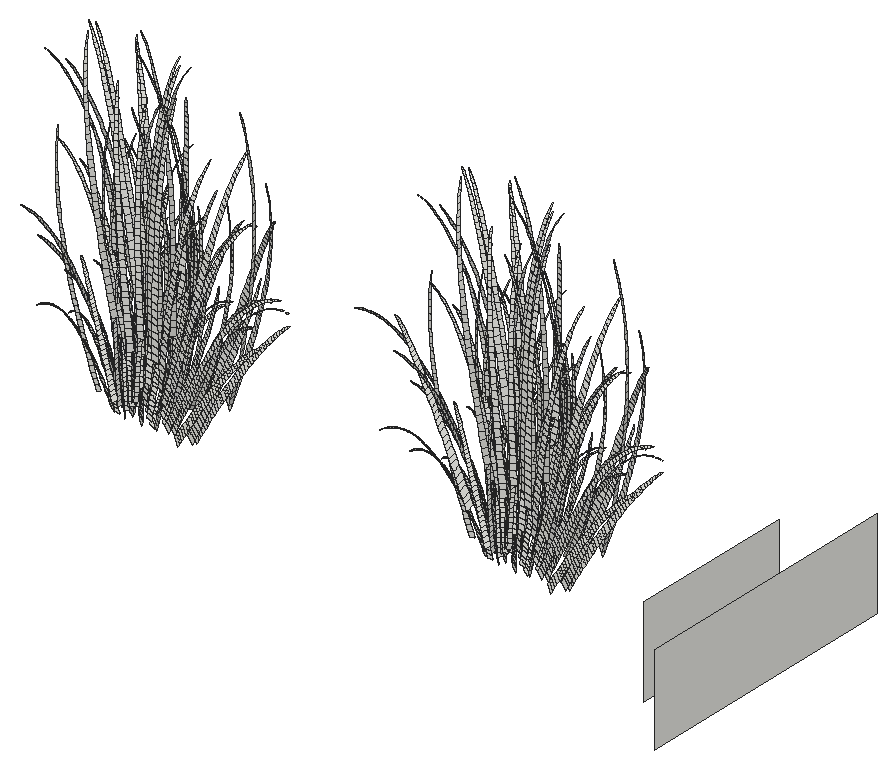
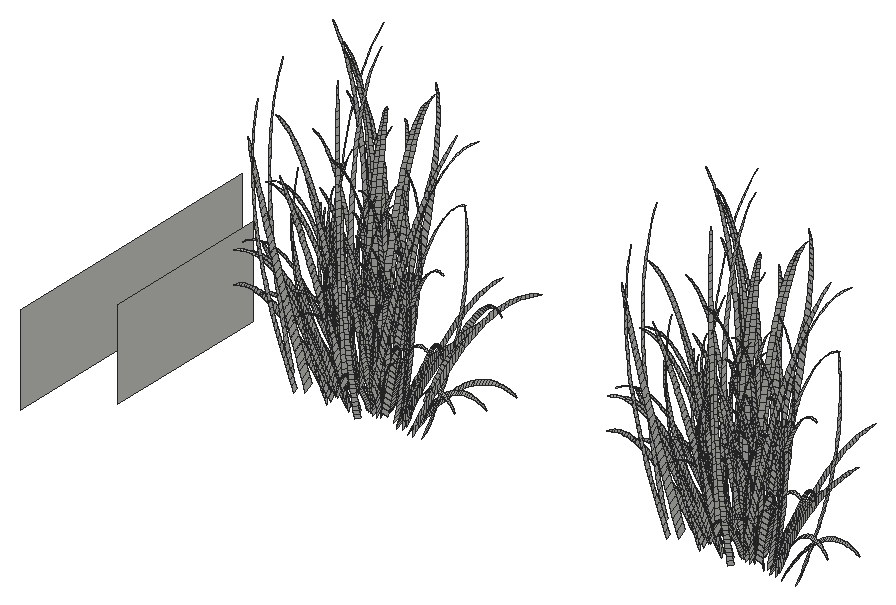
# SketchUp Ruby script. Lengths in inches.
U = 1.inch
M = Sketchup.active_model
def pt(a) = Geom::Point3d.new(a.map { |v| v * U })
def face(e, loops, mat)
  f = e.add_face(loops[0].map { |a| pt(a) })
  loops[1..].each { |l| e.add_face(l.map { |a| pt(a) }).erase! }
  f.material = f.back_material = mat if mat
  f
end
# faces: each face lists its corners as indices into pts; further lists are holes
def faces(e, pts, list, mat = nil) = list.each { |f| face(e, (f[0].is_a?(Array) ? f : [f]).map { |l| l.map { |i| pts[i] } }, mat) }
# xy, xz, yz: faces in a plane at the given z, y or x. An outline is a flat list of corners, or four numbers for a rectangle; further outlines are holes
def ring(l) = l.size == 4 ? [[l[0], l[1]], [l[2], l[1]], [l[2], l[3]], [l[0], l[3]]] : l.each_slice(2).to_a
def flat(e, list, mat, &to3) = list.each { |f| face(e, (f[0].is_a?(Array) ? f : [f]).map { |l| ring(l).map { |u, v| to3.(u, v) } }, mat) }
def xy(e, z, list, mat = nil) = flat(e, list, mat) { |x, y| [x, y, z] }
def xz(e, y, list, mat = nil) = flat(e, list, mat) { |x, z| [x, y, z] }
def yz(e, x, list, mat = nil) = flat(e, list, mat) { |y, z| [x, y, z] }
def lines(e, pts, list) = list.each { |a, b| e.add_line(pt(pts[a]), pt(pts[b])) }
# prism: a flat outline (further loops are holes) pulled along v
def prism(e, loops, v, mat = nil)
  f = face(e, loops, mat); d = Geom::Vector3d.new(v.map { |x| x * U })
  f.pushpull(f.normal.samedirection?(d) ? d.length : -d.length)
end
def box(e, o, s, mat = nil) = prism(e, [[o, [o[0] + s[0], o[1], o[2]], [o[0] + s[0], o[1] + s[1], o[2]], [o[0], o[1] + s[1], o[2]]]], [0, 0, s[2]], mat)
def at(x, y, z, deg = 0) = Geom::Transformation.translation(pt([x, y, z])) * Geom::Transformation.rotation(ORIGIN, Z_AXIS, deg.degrees)
def axes(o, x, y, z) = Geom::Transformation.new([*x, 0, *y, 0, *z, 0, *pt(o).to_a, 1])
def part(name) = M.definitions.add(name)
# library, detail: a bought-in or finely detailed component or shape, given as its bounding box
def library(name, o, s) = part(name).tap { |d| box(d.entities, o, s) }
def detail(e, o, s) = box(e.add_group.entities, o, s)
def put(e, d, t, mat = nil) = e.add_instance(d, t).tap { |i| i.material = mat if mat }
def group(e, t, mat = nil) = e.add_group.tap { |g| g.transformation = t; g.material = mat if mat }.entities
root = M.entities
c1 = part("fur_instance\#8")
p = [[-0.25,1.49,0.03],[0.25,-1.49,-0.03],[0.44,-1.47,1.51],[-0.05,1.47,1.57],[0.65,-1.44,3.05],[0.16,1.45,3.11],
  [0.86,-1.42,4.59],[0.38,1.44,4.65],[1.1,-1.39,6.13],[0.62,1.43,6.18],[1.34,-1.35,7.66],[0.875,1.42,7.72],
  [1.6,-1.32,9.19],[1.14,1.41,9.25],[1.88,-1.28,10.72],[1.43,1.41,10.78],[2.18,-1.24,12.25],[1.73,1.41,12.3],
  [2.49,-1.19,13.77],[2.05,1.41,13.82],[2.83,-1.15,15.29],[2.4,1.41,15.34],[3.18,-1.09,16.8],[2.76,1.42,16.85],
  [3.56,-1.03,18.31],[3.14,1.43,18.35],[3.96,-0.97,19.81],[3.55,1.44,19.85],[4.38,-0.91,21.3],[3.99,1.46,21.35],
  [4.84,-0.83,22.78],[4.45,1.48,22.83],[5.32,-0.76,24.26],[4.93,1.51,24.31],[5.82,-0.67,25.73],[5.45,1.54,25.77],
  [6.36,-0.59,27.18],[6,1.57,27.23],[6.93,-0.49,28.625],[6.58,1.61,28.67],[7.54,-0.39,30.05],[7.19,1.66,30.1],
  [8.18,-0.28,31.47],[7.84,1.71,31.51],[8.85,-0.16,32.86],[8.53,1.77,32.9],[9.57,-0.04,34.24],[9.25,1.83,34.27],
  [10.32,0.09,35.59],[10.02,1.9,35.625],[11.12,0.23,36.92],[10.82,1.97,36.95],[11.95,0.38,38.22],[11.67,2.06,38.25],
  [12.84,0.54,39.49],[12.57,2.14,39.52],[13.76,0.71,40.73],[13.51,2.24,40.76],[14.73,0.89,41.93],[14.49,2.34,41.95],
  [15.75,1.08,43.09],[15.52,2.45,43.11],[16.82,1.28,44.2],[16.6,2.5625,44.23],[17.93,1.5,45.27],[17.73,2.68,45.29],
  [19.08,1.73,46.28],[18.9,2.81,46.3],[20.29,1.97,47.24],[20.125,2.93,47.26],[21.53,2.22,48.13],[21.39,3.0625,48.15],
  [22.82,2.5,48.96],[22.7,3.1875,48.98],[24.14,2.8125,49.72],[24.06,3.3,49.73],[25.48,3.27,50.41]]
faces(c1.entities,p,[[0,1,2,3],[3,2,4,5],[5,4,6,7],[7,6,8,9],[9,8,10,11],[11,10,12,13],[13,12,14,15],[15,14,16,17],
  [17,16,18,19],[19,18,20,21],[21,20,22,23],[23,22,24,25],[25,24,26,27],[27,26,28,29],[29,28,30,31],[31,30,32,33],
  [33,32,34,35],[35,34,36,37],[37,36,38,39],[39,38,40,41],[41,40,42,43],[43,42,44,45],[45,44,46,47],[47,46,48,49],
  [49,48,50,51],[51,50,52,53],[53,52,54,55],[55,54,56,57],[57,56,58,59],[59,58,60,61],[61,60,62,63],[63,62,64,65],
  [65,64,66,67],[67,66,68,69],[69,68,70,71],[71,70,72,73],[73,72,74,75],[75,74,76]])
yz(root,230.42,[[60.29,0,79.88,10.375]])
yz(root,236.6875,[[54.02,0,86.15,10.375]])
put(root,c1,axes([166.59,68.19,3.78],[-0.15815,0.00988,0.0597],[0.01239,-0.13945,0.21255],[0.01922,0.06125,0.28145]))
put(root,c1,axes([209.9,68.19,3.78],[-0.15815,0.00988,0.0597],[0.01239,-0.13945,0.21255],[0.01922,0.06125,0.28145]))
put(root,c1,axes([160.72,70.96,3.6],[-0.1218,-0.13361,-0.0921],[0.11484,-0.14709,0.28095],[-0.12602,0.02393,0.36414]))
put(root,c1,axes([204.03,70.96,3.6],[-0.1218,-0.13361,-0.0921],[0.11484,-0.14709,0.28095],[-0.12602,0.02393,0.36414]))
put(root,c1,axes([166.42,68.81,10.79],[0.06704,0.21243,0.03183],[-0.23851,0.07708,0.05394],[0.01333,-0.07138,0.55186]))
put(root,c1,axes([209.73,68.81,10.79],[0.06704,0.21243,0.03183],[-0.23851,0.07708,0.05394],[0.01333,-0.07138,0.55186]))
put(root,c1,axes([168.57,71.8,10.04],[-0.21942,-0.09635,0.15751],[0.11362,-0.22061,0.00466],[0.05601,-0.02476,0.54483]))
put(root,c1,axes([211.88,71.8,10.04],[-0.21942,-0.09635,0.15751],[0.11362,-0.22061,0.00466],[0.05601,-0.02476,0.54483]))
put(root,c1,axes([162.28,69.1,10.41],[-0.01349,0.22403,0.09768],[-0.24396,0.034,-0.14422],[-0.06912,-0.0865,0.54108]))
put(root,c1,axes([205.59,69.1,10.41],[-0.01349,0.22403,0.09768],[-0.24396,0.034,-0.14422],[-0.06912,-0.0865,0.54108]))
put(root,c1,axes([166.99,68.57,9.44],[0.01128,0.21113,0.01155],[-0.2291,0.02553,0.05014],[0.01651,-0.05502,0.51224]))
put(root,c1,axes([210.3,68.57,9.44],[0.01128,0.21113,0.01155],[-0.2291,0.02553,0.05014],[0.01651,-0.05502,0.51224]))
put(root,c1,axes([168.19,69.84,1.93],[-0.03747,-0.12843,0.29203],[0.15407,-0.08219,-0.0652],[0.07562,0.07004,0.25518]))
put(root,c1,axes([211.5,69.84,1.93],[-0.03747,-0.12843,0.29203],[0.15407,-0.08219,-0.0652],[0.07562,0.07004,0.25518]))
put(root,c1,axes([164.09,68.6875,9.46],[-0.05249,0.21081,0.00883],[-0.2212,-0.0235,-0.05439],[-0.02833,-0.05377,0.50988]))
put(root,c1,axes([207.4,68.6875,9.46],[-0.05249,0.21081,0.00883],[-0.2212,-0.0235,-0.05439],[-0.02833,-0.05377,0.50988]))
put(root,c1,axes([163.61,67.75,4.02],[0.05338,0.14377,-0.04693],[-0.14103,0.06373,-0.16463],[-0.0677,0.01402,0.32804]))
put(root,c1,axes([206.93,67.75,4.02],[0.05338,0.14377,-0.04693],[-0.14103,0.06373,-0.16463],[-0.0677,0.01402,0.32804]))
put(root,c1,axes([165.86,69.22,11.18],[0.09204,0.20501,0.03679],[-0.23374,0.09978,0.05402],[0.01033,-0.07544,0.55902]))
put(root,c1,axes([209.18,69.22,11.18],[0.09204,0.20501,0.03679],[-0.23374,0.09978,0.05402],[0.01033,-0.07544,0.55902]))
put(root,c1,axes([167.68,68.6,8],[0.05117,0.19348,-0.04619],[-0.20175,0.05612,0.13032],[0.05644,-0.043,0.46253]))
put(root,c1,axes([210.99,68.6,8],[0.05117,0.19348,-0.04619],[-0.20175,0.05612,0.13032],[0.05644,-0.043,0.46253]))
put(root,c1,axes([163,69.78,7.8],[-0.20159,0.0718,-0.13723],[-0.04865,-0.19336,0.01671],[-0.06325,-0.01861,0.46524]))
put(root,c1,axes([206.31,69.78,7.8],[-0.20159,0.0718,-0.13723],[-0.04865,-0.19336,0.01671],[-0.06325,-0.01861,0.46524]))
put(root,c1,axes([164.45,68.42,4.45],[0.14782,0.0607,0.01728],[-0.06736,0.14608,-0.17165],[-0.04658,0.03213,0.33667]))
put(root,c1,axes([207.76,68.42,4.45],[0.14782,0.0607,0.01728],[-0.06736,0.14608,-0.17165],[-0.04658,0.03213,0.33667]))
put(root,c1,axes([162.89,69.4,2.0625],[-0.13656,-0.07352,-0.06681],[0.04427,-0.12761,0.28622],[-0.09439,0.0724,0.24805]))
put(root,c1,axes([206.2,69.4,2.0625],[-0.13656,-0.07352,-0.06681],[0.04427,-0.12761,0.28622],[-0.09439,0.0724,0.24805]))
put(root,c1,axes([167.04,67.71,3.85],[-0.04536,0.14528,-0.12173],[-0.14819,-0.02558,0.10276],[0.0266,0.02828,0.3139]))
put(root,c1,axes([210.35,67.71,3.85],[-0.04536,0.14528,-0.12173],[-0.14819,-0.02558,0.10276],[0.0266,0.02828,0.3139]))
put(root,c1,axes([165.85,69.48,5.74],[0.18587,-0.039,0.02017],[0.0261,0.16941,-0.18858],[-0.00202,0.04384,0.37494]))
put(root,c1,axes([209.16,69.48,5.74],[0.18587,-0.039,0.02017],[0.0261,0.16941,-0.18858],[-0.00202,0.04384,0.37494]))
put(root,c1,axes([164.71,68.13,4.21],[-0.10713,0.11469,-0.16211],[-0.11423,-0.10051,0.03718],[-0.0449,0.03097,0.32456]))
put(root,c1,axes([208.02,68.13,4.21],[-0.10713,0.11469,-0.16211],[-0.11423,-0.10051,0.03718],[-0.0449,0.03097,0.32456]))
put(root,c1,axes([164.64,71.86,11.71],[0.25389,-0.06297,0.01758],[0.0429,0.23535,-0.03956],[-0.01113,-0.0353,0.57531]))
put(root,c1,axes([207.95,71.86,11.71],[0.25389,-0.06297,0.01758],[0.0429,0.23535,-0.03956],[-0.01113,-0.0353,0.57531]))
put(root,c1,axes([166.56,69.88,8.16],[-0.20845,0.0617,0.05447],[-0.04632,-0.1966,0.1192],[0.03082,-0.00313,0.46484]))
put(root,c1,axes([209.87,69.88,8.16],[-0.20845,0.0617,0.05447],[-0.04632,-0.1966,0.1192],[0.03082,-0.00313,0.46484]))
put(root,c1,axes([163.78,69.95,3.18],[0.12753,-0.09379,0.22491],[0.10527,0.1265,-0.10063],[-0.06372,0.06207,0.3109]))
put(root,c1,axes([207.09,69.95,3.18],[0.12753,-0.09379,0.22491],[0.10527,0.1265,-0.10063],[-0.06372,0.06207,0.3109]))
put(root,c1,axes([161.48,70.53,2.85],[-0.12578,-0.12091,-0.0564],[0.08033,-0.12818,0.33188],[-0.12725,0.06361,0.28183]))
put(root,c1,axes([204.79,70.53,2.85],[-0.12578,-0.12091,-0.0564],[0.08033,-0.12818,0.33188],[-0.12725,0.06361,0.28183]))
put(root,c1,axes([164.09,68.82,2.88],[0.15191,0.00864,0.09894],[-0.00116,0.14441,-0.20359],[-0.05853,0.05702,0.28561]))
put(root,c1,axes([207.4,68.82,2.88],[0.15191,0.00864,0.09894],[-0.00116,0.14441,-0.20359],[-0.05853,0.05702,0.28561]))
put(root,c1,axes([169.9,68.1,2.31],[0.00579,0.17068,-0.16321],[-0.12957,0.03754,0.26919],[0.12935,0.00849,0.26276]))
put(root,c1,axes([213.21,68.1,2.31],[0.00579,0.17068,-0.16321],[-0.12957,0.03754,0.26919],[0.12935,0.00849,0.26276]))
put(root,c1,axes([163.7,69,3.28],[0.15072,0.0136,0.13727],[-0.00409,0.15385,-0.193],[-0.07769,0.04892,0.29677]))
put(root,c1,axes([207.01,69,3.28],[0.15072,0.0136,0.13727],[-0.00409,0.15385,-0.193],[-0.07769,0.04892,0.29677]))
put(root,c1,axes([165.41,69.77,2.5],[-0.01699,-0.12732,0.27857],[0.16448,-0.01291,0.05595],[-0.02464,0.09551,0.24356]))
put(root,c1,axes([208.72,69.77,2.5],[-0.01699,-0.12732,0.27857],[0.16448,-0.01291,0.05595],[-0.02464,0.09551,0.24356]))
put(root,c1,axes([163.29,71.28,8.1],[0.21265,-0.06804,0.11906],[0.05038,0.20319,-0.07151],[-0.05071,-0.00134,0.48262]))
put(root,c1,axes([206.6,71.28,8.1],[0.21265,-0.06804,0.11906],[0.05038,0.20319,-0.07151],[-0.05071,-0.00134,0.48262]))
put(root,c1,axes([168.62,69.17,4.39],[-0.16864,0.05731,0.14747],[-0.02228,-0.16808,0.21885],[0.0836,0.03526,0.33224]))
put(root,c1,axes([211.93,69.17,4.39],[-0.16864,0.05731,0.14747],[-0.02228,-0.16808,0.21885],[0.0836,0.03526,0.33224]))
put(root,c1,axes([168.22,70.15,2.62],[0.14782,-0.11273,0.00048],[0.0732,0.11159,-0.31128],[0.07867,0.07287,0.26546]))
put(root,c1,axes([211.53,70.15,2.62],[0.14782,-0.11273,0.00048],[0.0732,0.11159,-0.31128],[0.07867,0.07287,0.26546]))
put(root,c1,axes([203.24,70.74,2.83],[-0.13408,-0.01944,-0.33055],[0.01755,-0.20151,0.16145],[-0.16419,0.01714,0.30229]))
put(root,c1,axes([158.8125,70.72,2.61],[0.14067,-0.04522,0.3848],[0.02544,0.20918,-0.05629],[-0.17357,0.01812,0.31957]))
put(root,c1,axes([202.125,70.72,2.61],[0.14067,-0.04522,0.3848],[0.02544,0.20918,-0.05629],[-0.17357,0.01812,0.31957]))
put(root,c1,axes([161.23,69.8,1.9],[-0.1289,0.01316,-0.29885],[-0.02366,-0.17656,0.13341],[-0.13753,0.03975,0.27153]))
put(root,c1,axes([204.54,69.8,1.9],[-0.1289,0.01316,-0.29885],[-0.02366,-0.17656,0.13341],[-0.13753,0.03975,0.27153]))
put(root,c1,axes([166.87,70.22,2.09],[0.01055,-0.13508,0.28615],[0.17058,-0.02073,-0.06684],[0.02674,0.09288,0.2522]))
put(root,c1,axes([210.18,70.22,2.09],[0.01055,-0.13508,0.28615],[0.17058,-0.02073,-0.06684],[0.02674,0.09288,0.2522]))
put(root,c1,axes([168.71,68.97,6.82],[0.08157,0.17825,-0.15725],[-0.17491,0.09532,0.15482],[0.08885,-0.01806,0.42132]))
put(root,c1,axes([212.02,68.97,6.82],[0.08157,0.17825,-0.15725],[-0.17491,0.09532,0.15482],[0.08885,-0.01806,0.42132]))
put(root,c1,axes([164.16,69.31,3.95],[0.16194,-0.0082,0.12991],[0.01706,0.15486,-0.20493],[-0.06274,0.06113,0.30616]))
put(root,c1,axes([207.48,69.31,3.95],[0.16194,-0.0082,0.12991],[0.01706,0.15486,-0.20493],[-0.06274,0.06113,0.30616]))
put(root,c1,axes([165.63,69.43,7.59],[-0.17716,0.11278,-0.05906],[-0.10338,-0.15992,0.10796],[-0.00363,0.01008,0.44244]))
put(root,c1,axes([208.94,69.43,7.59],[-0.17716,0.11278,-0.05906],[-0.10338,-0.15992,0.10796],[-0.00363,0.01008,0.44244]))
put(root,c1,axes([165.2,68.12,4.8125],[0.03769,0.14922,-0.14278],[-0.15939,0.04231,-0.09138],[-0.03216,0.03689,0.33298]))
put(root,c1,axes([208.51,68.12,4.8125],[0.03769,0.14922,-0.14278],[-0.15939,0.04231,-0.09138],[-0.03216,0.03689,0.33298]))
put(root,c1,axes([165.33,68.34,3.55],[0.13054,0.07134,-0.09742],[-0.08675,0.11604,-0.1956],[-0.0202,0.06504,0.27821]))
put(root,c1,axes([208.64,68.34,3.55],[0.13054,0.07134,-0.09742],[-0.08675,0.11604,-0.1956],[-0.0202,0.06504,0.27821]))
put(root,c1,axes([162.27,69.02,2.35],[-0.11086,0.06293,-0.29386],[-0.07533,-0.1452,0.07106],[-0.11428,0.05713,0.25311]))
put(root,c1,axes([205.58,69.02,2.35],[-0.11086,0.06293,-0.29386],[-0.07533,-0.1452,0.07106],[-0.11428,0.05713,0.25311]))
put(root,c1,axes([167.87,71.14,3.6],[-0.10724,-0.12303,0.26265],[0.15657,-0.12402,0.06415],[0.04661,0.06574,0.34387]))
put(root,c1,axes([211.18,71.14,3.6],[-0.10724,-0.12303,0.26265],[0.15657,-0.12402,0.06415],[0.04661,0.06574,0.34387]))
put(root,c1,axes([166.81,68.99,2.28],[-0.15615,0.01011,0.08042],[0.021,-0.12557,0.25868],[0.02465,0.08562,0.2325]))
put(root,c1,axes([210.12,68.99,2.28],[-0.15615,0.01011,0.08042],[0.021,-0.12557,0.25868],[0.02465,0.08562,0.2325]))
put(root,c1,axes([162.14,70.21,2.26],[0.12181,-0.05572,0.30355],[0.07119,0.15699,-0.09562],[-0.1203,0.06014,0.26644]))
put(root,c1,axes([205.46,70.21,2.26],[0.12181,-0.05572,0.30355],[0.07119,0.15699,-0.09562],[-0.1203,0.06014,0.26644]))
put(root,c1,axes([166.81,69.51,6.125],[-0.18299,0.07424,0.021],[-0.05602,-0.16634,0.19558],[0.03285,0.03492,0.38761]))
put(root,c1,axes([210.12,69.51,6.125],[-0.18299,0.07424,0.021],[-0.05602,-0.16634,0.19558],[0.03285,0.03492,0.38761]))
put(root,c1,axes([164.8,69.36,9.17],[-0.02533,0.21082,-0.03246],[-0.22123,-0.00286,-0.02372],[-0.01766,-0.03271,0.49841]))
put(root,c1,axes([208.11,69.36,9.17],[-0.02533,0.21082,-0.03246],[-0.22123,-0.00286,-0.02372],[-0.01766,-0.03271,0.49841]))
put(root,c1,axes([166.96,71.25,10.99],[-0.23935,0.06874,0.11641],[-0.05487,-0.22915,0.10476],[0.05566,-0.0246,0.54145]))
put(root,c1,axes([210.27,71.25,10.99],[-0.23935,0.06874,0.11641],[-0.05487,-0.22915,0.10476],[0.05566,-0.0246,0.54145]))
put(root,c1,axes([166.01,68.87,6.65],[-0.04271,0.18174,-0.10347],[-0.18723,-0.02484,0.051],[0.00749,0.00721,0.41447]))
put(root,c1,axes([209.32,68.87,6.65],[-0.04271,0.18174,-0.10347],[-0.18723,-0.02484,0.051],[0.00749,0.00721,0.41447]))
put(root,c1,axes([162.1,68.9,3.52],[-0.0676,0.15738,-0.2157],[-0.13135,-0.07732,-0.14677],[-0.1112,0.02111,0.32133]))
put(root,c1,axes([205.41,68.9,3.52],[-0.0676,0.15738,-0.2157],[-0.13135,-0.07732,-0.14677],[-0.1112,0.02111,0.32133]))
put(root,c1,axes([164.95,69.14,2.12],[-0.14803,0.01323,-0.11537],[-0.03176,-0.12328,0.24366],[-0.04653,0.08668,0.23028]))
put(root,c1,axes([208.26,69.14,2.12],[-0.14803,0.01323,-0.11537],[-0.03176,-0.12328,0.24366],[-0.04653,0.08668,0.23028]))
put(root,c1,axes([169.92,69.47,2.6875],[-0.14434,0.09377,0.17872],[-0.03919,-0.15638,0.28066],[0.124,0.03453,0.28007]))
put(root,c1,axes([213.23,69.47,2.6875],[-0.14434,0.09377,0.17872],[-0.03919,-0.15638,0.28066],[0.124,0.03453,0.28007]))
put(root,c1,axes([169.51,69.52,5.22],[0.1044,0.14559,-0.25751],[-0.13502,0.13555,0.13946],[0.11942,-0.00409,0.36287]))
put(root,c1,axes([212.82,69.52,5.22],[0.1044,0.14559,-0.25751],[-0.13502,0.13555,0.13946],[0.11942,-0.00409,0.36287]))
put(root,c1,axes([169.11,69.59,8.58],[0.01228,0.22259,-0.04839],[-0.21245,0.01489,0.2439],[0.10506,-0.04029,0.46949]))
put(root,c1,axes([212.42,69.59,8.58],[0.01228,0.22259,-0.04839],[-0.21245,0.01489,0.2439],[0.10506,-0.04029,0.46949]))
put(root,c1,axes([164.97,70.2,2.65],[0.1046,-0.10479,0.24905],[0.1356,0.08115,-0.15676],[-0.02552,0.09892,0.25225]))
put(root,c1,axes([208.28,70.2,2.65],[0.1046,-0.10479,0.24905],[0.1356,0.08115,-0.15676],[-0.02552,0.09892,0.25225]))
put(root,c1,axes([168.43,69.5625,4.06],[-0.15929,0.09132,0.09708],[-0.05737,-0.15132,0.24406],[0.08321,0.03509,0.33068]))
put(root,c1,axes([211.75,69.5625,4.06],[-0.15929,0.09132,0.09708],[-0.05737,-0.15132,0.24406],[0.08321,0.03509,0.33068]))
put(root,c1,axes([162.04,72.36,4.41],[0.01665,-0.19186,0.25247],[0.18867,0.0288,0.15737],[-0.09759,0.06145,0.3728]))
put(root,c1,axes([205.36,72.36,4.41],[0.01665,-0.19186,0.25247],[0.18867,0.0288,0.15737],[-0.09759,0.06145,0.3728]))
put(root,c1,axes([167.94,69.15,2.65],[-0.15229,0.06835,0.08842],[-0.02287,-0.13137,0.27682],[0.07344,0.06802,0.24782]))
put(root,c1,axes([211.26,69.15,2.65],[-0.15229,0.06835,0.08842],[-0.02287,-0.13137,0.27682],[0.07344,0.06802,0.24782]))
put(root,c1,axes([168.26,68.76,2.78],[-0.11038,0.13094,-0.01587],[-0.09023,-0.08182,0.28993],[0.09271,0.05046,0.24619]))
put(root,c1,axes([211.57,68.76,2.78],[-0.11038,0.13094,-0.01587],[-0.09023,-0.08182,0.28993],[0.09271,0.05046,0.24619]))
put(root,c1,axes([166.77,69.33,3.7],[0.1552,0.04284,-0.14088],[-0.07244,0.14474,-0.19228],[0.02075,0.06614,0.30388]))
put(root,c1,axes([210.09,69.33,3.7],[0.1552,0.04284,-0.14088],[-0.07244,0.14474,-0.19228],[0.02075,0.06614,0.30388]))
put(root,c1,axes([163.51,70.96,11.74],[-0.19599,0.17659,-0.04249],[-0.16606,-0.16516,-0.03794],[-0.03174,-0.0516,0.57661]))
put(root,c1,axes([206.82,70.96,11.74],[-0.19599,0.17659,-0.04249],[-0.16606,-0.16516,-0.03794],[-0.03174,-0.0516,0.57661]))
put(root,c1,axes([164.72,70.02,7.95],[0.1688,0.10784,-0.0329],[-0.12628,0.17185,-0.12449],[-0.0276,0.0088,0.45819]))
put(root,c1,axes([208.04,70.02,7.95],[0.1688,0.10784,-0.0329],[-0.12628,0.17185,-0.12449],[-0.0276,0.0088,0.45819]))
put(root,c1,axes([170.4,69.51,2.08],[-0.08133,0.16944,0.041],[-0.11353,-0.08181,0.33645],[0.13926,0.00914,0.28291]))
put(root,c1,axes([213.72,69.51,2.08],[-0.08133,0.16944,0.041],[-0.11353,-0.08181,0.33645],[0.13926,0.00914,0.28291]))
put(root,c1,axes([161.51,70.27,7.2],[0.12687,0.1431,0.11306],[-0.15006,0.15928,-0.20805],[-0.10892,-0.0144,0.44372]))
put(root,c1,axes([204.82,70.27,7.2],[0.12687,0.1431,0.11306],[-0.15006,0.15928,-0.20805],[-0.10892,-0.0144,0.44372]))
put(root,c1,axes([163.66,68.76,3.16],[-0.00457,0.15131,-0.19037],[-0.14827,-0.01393,-0.13436],[-0.07643,0.04813,0.29198]))
put(root,c1,axes([206.97,68.76,3.16],[-0.00457,0.15131,-0.19037],[-0.14827,-0.01393,-0.13436],[-0.07643,0.04813,0.29198]))
put(root,c1,axes([161.375,71.55,3.72],[0.1591,-0.07433,0.27972],[0.07325,0.17912,-0.08368],[-0.11229,0.04342,0.36287]))
put(root,c1,axes([204.6875,71.55,3.72],[0.1591,-0.07433,0.27972],[0.07325,0.17912,-0.08368],[-0.11229,0.04342,0.36287]))
put(root,c1,axes([167.35,70.95,7.05],[0.2064,0.00506,-0.149],[-0.0314,0.20396,-0.16093],[0.05385,0.02809,0.42994]))
put(root,c1,axes([210.66,70.95,7.05],[0.2064,0.00506,-0.149],[-0.0314,0.20396,-0.16093],[0.05385,0.02809,0.42994]))
put(root,c1,axes([167.43,69.43,4.6875],[-0.1523,0.1081,0.01181],[-0.08113,-0.12936,0.25496],[0.06382,0.04964,0.32324]))
put(root,c1,axes([210.74,69.43,4.6875],[-0.1523,0.1081,0.01181],[-0.08113,-0.12936,0.25496],[0.06382,0.04964,0.32324]))
put(root,c1,axes([164.07,70.72,3.07],[0.16515,-0.05448,0.15409],[0.06343,0.14946,-0.20076],[-0.0453,0.07156,0.32105]))
put(root,c1,axes([207.39,70.72,3.07],[0.16515,-0.05448,0.15409],[0.06343,0.14946,-0.20076],[-0.0453,0.07156,0.32105]))
put(root,c1,axes([163.36,69.79,3.47],[-0.13323,0.08202,-0.23675],[-0.08835,-0.14174,0.08371],[-0.08237,0.05187,0.31467]))
put(root,c1,axes([206.67,69.79,3.47],[-0.13323,0.08202,-0.23675],[-0.08835,-0.14174,0.08371],[-0.08237,0.05187,0.31467]))
put(root,c1,axes([167.14,71.84,5.42],[0.16589,-0.13509,0.0734],[0.11769,0.12965,-0.28034],[0.04996,0.07046,0.36857]))
put(root,c1,axes([210.45,71.84,5.42],[0.16589,-0.13509,0.0734],[0.11769,0.12965,-0.28034],[0.04996,0.07046,0.36857]))
put(root,c1,axes([169.4,70.89,4.3125],[0.18376,0.00291,-0.23488],[-0.03958,0.19621,-0.17283],[0.09238,0.03896,0.36714]))
put(root,c1,axes([212.71,70.89,4.3125],[0.18376,0.00291,-0.23488],[-0.03958,0.19621,-0.17283],[0.09238,0.03896,0.36714]))
put(root,c1,axes([168.5,70.99,3.73],[0.18658,-0.03164,-0.14855],[-0.00603,0.17961,-0.23275],[0.06904,0.0537,0.34969]))
put(root,c1,axes([211.81,70.99,3.73],[0.18658,-0.03164,-0.14855],[-0.00603,0.17961,-0.23275],[0.06904,0.0537,0.34969]))
put(root,c1,axes([169.57,71.46,2.72],[-0.14001,-0.05504,0.33454],[0.10116,-0.17879,0.10883],[0.11232,0.06113,0.29828]))
put(root,c1,axes([212.88,71.46,2.72],[-0.14001,-0.05504,0.33454],[0.10116,-0.17879,0.10883],[0.11232,0.06113,0.29828]))
put(root,c1,axes([202.21,70.33,5.8],[-0.11905,0.20326,-0.22454],[-0.13951,-0.10936,-0.26462],[-0.15957,-0.02537,0.41917]))
put(root,c1,axes([161.79,72.79,10.54],[-0.24661,-0.01011,-0.12308],[0.03558,-0.24626,0.10561],[-0.06805,-0.01098,0.55498]))
put(root,c1,axes([205.1,72.79,10.54],[-0.24661,-0.01011,-0.12308],[0.03558,-0.24626,0.10561],[-0.06805,-0.01098,0.55498]))
put(root,c1,axes([172.46,72.8,5.08],[-0.20751,-0.0154,0.34807],[0.03231,-0.24429,0.09326],[0.14695,-0.00503,0.44651]))
put(root,c1,axes([215.78,72.8,5.08],[-0.20751,-0.0154,0.34807],[0.03231,-0.24429,0.09326],[0.14695,-0.00503,0.44651]))
put(root,c1,axes([165.74,73.46,7.625],[0.08686,-0.20683,0.21585],[0.21659,0.06277,-0.09493],[-0.00252,0.05451,0.46618]))
put(root,c1,axes([209.05,73.46,7.625],[0.08686,-0.20683,0.21585],[0.21659,0.06277,-0.09493],[-0.00252,0.05451,0.46618]))
put(root,c1,axes([163.51,71.36,11.57],[-0.19695,0.1732,-0.04859],[-0.16287,-0.16855,-0.01576],[-0.02749,-0.04327,0.57313]))
put(root,c1,axes([206.83,71.36,11.57],[-0.19695,0.1732,-0.04859],[-0.16287,-0.16855,-0.01576],[-0.02749,-0.04327,0.57313]))
put(root,c1,axes([162.19,70.27,2.78],[0.14298,0.02776,0.2221],[0.00324,0.16655,-0.23396],[-0.12194,0.06096,0.27007]))
put(root,c1,axes([205.5,70.27,2.78],[0.14298,0.02776,0.2221],[0.00324,0.16655,-0.23396],[-0.12194,0.06096,0.27007]))
put(root,c1,axes([200.9,73.83,4.96],[-0.16665,-0.10839,-0.24928],[0.10528,-0.22,0.26583],[-0.16455,0.00217,0.44452]))
put(root,c1,axes([166.5625,71.14,5.4375],[-0.20063,0.02155,0.04243],[-0.00141,-0.18611,0.19899],[0.01635,0.04322,0.40207]))
put(root,c1,axes([209.875,71.14,5.4375],[-0.20063,0.02155,0.04243],[-0.00141,-0.18611,0.19899],[0.01635,0.04322,0.40207]))
put(root,c1,axes([171.41,73.69,4.2],[-0.06693,-0.18459,0.37403],[0.17622,-0.13687,-0.1896],[0.15627,0.04352,0.35297]))
put(root,c1,axes([214.73,73.69,4.2],[-0.06693,-0.18459,0.37403],[0.17622,-0.13687,-0.1896],[0.15627,0.04352,0.35297]))
put(root,c1,axes([166.01,71.73,5.01],[0.16091,-0.11894,0.16216],[0.12315,0.12828,-0.22813],[-0.0007,0.08282,0.35694]))
put(root,c1,axes([209.32,71.73,5.01],[0.16091,-0.11894,0.16216],[0.12315,0.12828,-0.22813],[-0.0007,0.08282,0.35694]))
put(root,c1,axes([170.65,69.79,2.21],[-0.00334,0.19157,-0.16025],[-0.14373,0.02868,0.30995],[0.14337,0.00941,0.29124]))
put(root,c1,axes([213.96,69.79,2.21],[-0.00334,0.19157,-0.16025],[-0.14373,0.02868,0.30995],[0.14337,0.00941,0.29124]))
put(root,c1,axes([167.8,71.38,6.34],[-0.20765,0.04551,0.10452],[-0.02061,-0.19877,0.19268],[0.05382,0.02807,0.42972]))
put(root,c1,axes([211.11,71.38,6.34],[-0.20765,0.04551,0.10452],[-0.02061,-0.19877,0.19268],[0.05382,0.02807,0.42972]))
put(root,c1,axes([169.73,73.91,5.15],[0.12626,-0.20284,0.07113],[0.17291,0.09387,-0.32445],[0.10522,0.04438,0.41818]))
put(root,c1,axes([213.04,73.91,5.15],[0.12626,-0.20284,0.07113],[0.17291,0.09387,-0.32445],[0.10522,0.04438,0.41818]))
put(root,c1,axes([167.36,69.23,3.6],[0.03504,0.14333,-0.23786],[-0.16522,0.06024,0.03644],[0.04149,0.05851,0.30605]))
put(root,c1,axes([210.67,69.23,3.6],[0.03504,0.14333,-0.23786],[-0.16522,0.06024,0.03644],[0.04149,0.05851,0.30605]))
put(root,c1,axes([164.09,69.57,3.92],[0.12802,0.10582,-0.05497],[-0.1046,0.11656,-0.24012],[-0.0637,0.06206,0.31081]))
put(root,c1,axes([207.4,69.57,3.92],[0.12802,0.10582,-0.05497],[-0.1046,0.11656,-0.24012],[-0.0637,0.06206,0.31081]))
put(root,c1,axes([165.55,71.39,5.85],[-0.2047,0.01723,0.00593],[-0.00087,-0.18882,0.20676],[-0.00221,0.04782,0.40893]))
put(root,c1,axes([208.86,71.39,5.85],[-0.2047,0.01723,0.00593],[-0.00087,-0.18882,0.20676],[-0.00221,0.04782,0.40893]))
put(root,c1,axes([164.24,69.89,5.21],[-0.11141,0.14453,-0.18255],[-0.14786,-0.09923,0.0582],[-0.03635,0.0417,0.37637]))
put(root,c1,axes([207.55,69.89,5.21],[-0.11141,0.14453,-0.18255],[-0.14786,-0.09923,0.0582],[-0.03635,0.0417,0.37637]))
put(root,c1,axes([167.49,70.18,4.25],[-0.17132,0.08809,0.00001],[-0.06467,-0.14373,0.26091],[0.04498,0.06344,0.33183]))
put(root,c1,axes([210.8,70.18,4.25],[-0.17132,0.08809,0.00001],[-0.06467,-0.14373,0.26091],[0.04498,0.06344,0.33183]))
put(root,c1,axes([167.55,70.75,2.55],[-0.16842,0.00001,0.17613],[0.0504,-0.15213,0.25899],[0.055,0.08838,0.2682]))
put(root,c1,axes([210.86,70.75,2.55],[-0.16842,0.00001,0.17613],[0.0504,-0.15213,0.25899],[0.055,0.08838,0.2682]))
put(root,c1,axes([164.66,70.98,3.61],[-0.18524,0.01318,-0.044],[-0.00864,-0.16062,0.25477],[-0.0239,0.07696,0.32915]))
put(root,c1,axes([207.97,70.98,3.61],[-0.18524,0.01318,-0.044],[-0.00864,-0.16062,0.25477],[-0.0239,0.07696,0.32915]))
put(root,c1,axes([165.22,71.5,10.81],[-0.15522,0.19417,-0.03161],[-0.19201,-0.12962,0.02598],[-0.00591,-0.03393,0.55136]))
put(root,c1,axes([208.53,71.5,10.81],[-0.15522,0.19417,-0.03161],[-0.19201,-0.12962,0.02598],[-0.00591,-0.03393,0.55136]))
put(root,c1,axes([166.17,69.3,2.1],[-0.06121,0.11818,-0.24749],[-0.14799,-0.03414,0.11286],[0.00064,0.09094,0.23354]))
put(root,c1,axes([209.49,69.3,2.1],[-0.06121,0.11818,-0.24749],[-0.14799,-0.03414,0.11286],[0.00064,0.09094,0.23354]))
put(root,c1,axes([162.32,71.08,6.85],[-0.16212,0.13096,-0.2268],[-0.11678,-0.16208,0.00347],[-0.08971,0.01858,0.43465]))
put(root,c1,axes([205.64,71.08,6.85],[-0.16212,0.13096,-0.2268],[-0.11678,-0.16208,0.00347],[-0.08971,0.01858,0.43465]))
put(root,c1,axes([163.96,70.36,8.17],[0.03814,0.2015,-0.09604],[-0.21147,0.05412,-0.09289],[-0.03952,0.00488,0.47049]))
put(root,c1,axes([207.27,70.36,8.17],[0.03814,0.2015,-0.09604],[-0.21147,0.05412,-0.09289],[-0.03952,0.00488,0.47049]))
put(root,c1,axes([161.42,74.84,7.67],[-0.12046,-0.19753,0.07695],[0.20061,-0.12871,0.24478],[-0.08711,0.03599,0.49657]))
put(root,c1,axes([204.74,74.84,7.67],[-0.12046,-0.19753,0.07695],[0.20061,-0.12871,0.24478],[-0.08711,0.03599,0.49657]))
put(root,c1,axes([160.93,71.44,4.41],[0.17949,0.03208,0.20009],[-0.02216,0.19765,-0.22548],[-0.11594,0.04484,0.37468]))
put(root,c1,axes([204.24,71.44,4.41],[0.17949,0.03208,0.20009],[-0.02216,0.19765,-0.22548],[-0.11594,0.04484,0.37468]))
put(root,c1,axes([164.66,71.48,11.13],[-0.12955,0.21354,-0.0433],[-0.21401,-0.10243,0.0018],[-0.01549,-0.03509,0.55942]))
put(root,c1,axes([207.97,71.48,11.13],[-0.12955,0.21354,-0.0433],[-0.21401,-0.10243,0.0018],[-0.01549,-0.03509,0.55942]))
put(root,c1,axes([162.62,70.35,6.95],[0.00664,0.20286,-0.1262],[-0.19518,0.01818,-0.18229],[-0.08769,0.01816,0.42485]))
put(root,c1,axes([205.93,70.35,6.95],[0.00664,0.20286,-0.1262],[-0.19518,0.01818,-0.18229],[-0.08769,0.01816,0.42485]))
put(root,c1,axes([165.1875,72.47,2.95],[0.03807,-0.14827,0.33406],[0.19165,0.02974,-0.03379],[-0.02912,0.11286,0.28781]))
put(root,c1,axes([208.5,72.47,2.95],[0.03807,-0.14827,0.33406],[0.19165,0.02974,-0.03379],[-0.02912,0.11286,0.28781]))
put(root,c1,axes([163.6,69.77,2.21],[0.10395,0.11836,-0.12851],[-0.11439,0.07411,-0.26217],[-0.07351,0.08501,0.2481]))
